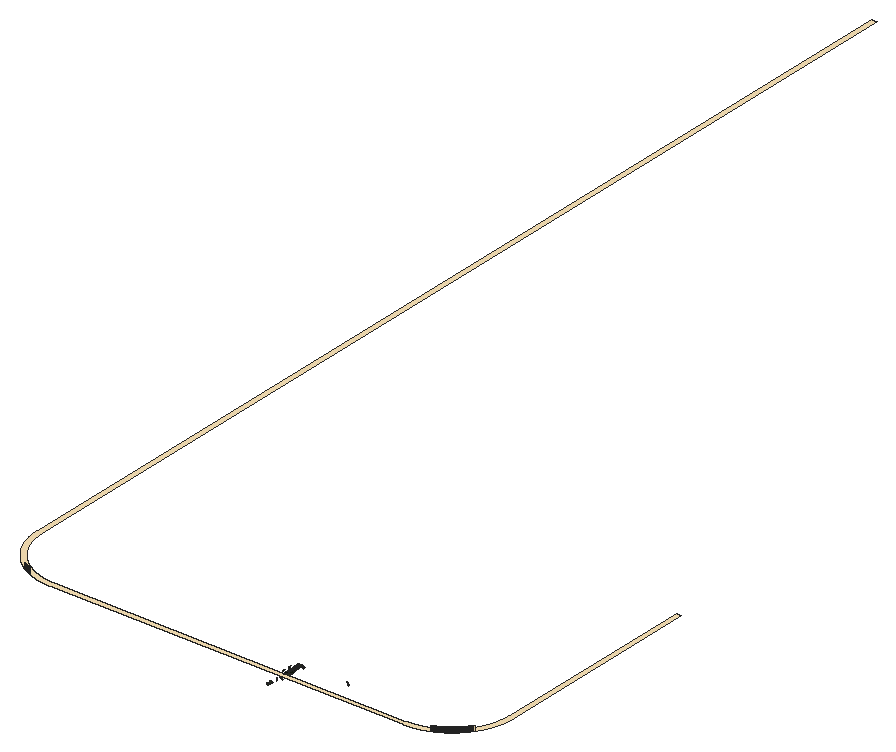
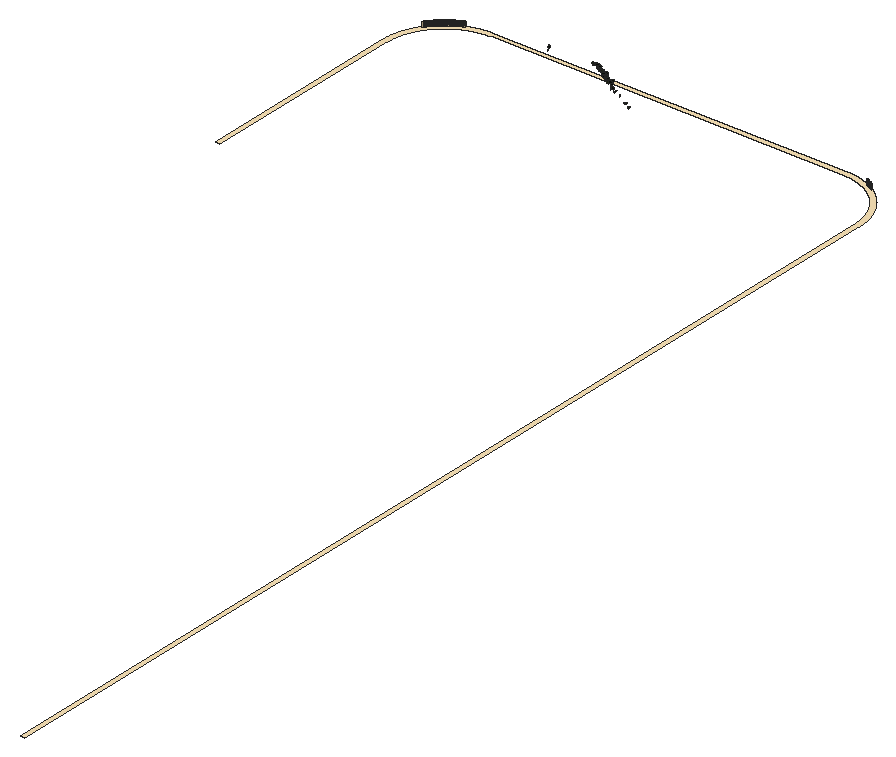
# SketchUp Ruby script. Lengths in inches.
U = 1.inch
M = Sketchup.active_model
def pt(a) = Geom::Point3d.new(a.map { |v| v * U })
def face(e, loops, mat)
  f = e.add_face(loops[0].map { |a| pt(a) })
  loops[1..].each { |l| e.add_face(l.map { |a| pt(a) }).erase! }
  f.material = f.back_material = mat if mat
  f
end
# faces: each face lists its corners as indices into pts; further lists are holes
def faces(e, pts, list, mat = nil) = list.each { |f| face(e, (f[0].is_a?(Array) ? f : [f]).map { |l| l.map { |i| pts[i] } }, mat) }
# xy, xz, yz: faces in a plane at the given z, y or x. An outline is a flat list of corners, or four numbers for a rectangle; further outlines are holes
def ring(l) = l.size == 4 ? [[l[0], l[1]], [l[2], l[1]], [l[2], l[3]], [l[0], l[3]]] : l.each_slice(2).to_a
def flat(e, list, mat, &to3) = list.each { |f| face(e, (f[0].is_a?(Array) ? f : [f]).map { |l| ring(l).map { |u, v| to3.(u, v) } }, mat) }
def xy(e, z, list, mat = nil) = flat(e, list, mat) { |x, y| [x, y, z] }
def xz(e, y, list, mat = nil) = flat(e, list, mat) { |x, z| [x, y, z] }
def yz(e, x, list, mat = nil) = flat(e, list, mat) { |y, z| [x, y, z] }
def lines(e, pts, list) = list.each { |a, b| e.add_line(pt(pts[a]), pt(pts[b])) }
# prism: a flat outline (further loops are holes) pulled along v
def prism(e, loops, v, mat = nil)
  f = face(e, loops, mat); d = Geom::Vector3d.new(v.map { |x| x * U })
  f.pushpull(f.normal.samedirection?(d) ? d.length : -d.length)
end
def box(e, o, s, mat = nil) = prism(e, [[o, [o[0] + s[0], o[1], o[2]], [o[0] + s[0], o[1] + s[1], o[2]], [o[0], o[1] + s[1], o[2]]]], [0, 0, s[2]], mat)
def at(x, y, z, deg = 0) = Geom::Transformation.translation(pt([x, y, z])) * Geom::Transformation.rotation(ORIGIN, Z_AXIS, deg.degrees)
def axes(o, x, y, z) = Geom::Transformation.new([*x, 0, *y, 0, *z, 0, *pt(o).to_a, 1])
def part(name) = M.definitions.add(name)
# library, detail: a bought-in or finely detailed component or shape, given as its bounding box
def library(name, o, s) = part(name).tap { |d| box(d.entities, o, s) }
def detail(e, o, s) = box(e.add_group.entities, o, s)
def put(e, d, t, mat = nil) = e.add_instance(d, t).tap { |i| i.material = mat if mat }
def group(e, t, mat = nil) = e.add_group.tap { |g| g.transformation = t; g.material = mat if mat }.entities
root = M.entities
M.materials.add("1026 AP 7946 SUNNY SIDE UP").color = [254, 231, 186]
M.materials.add("efeu1").color = [18, 25, 13]
M.materials.add("efeu2").color = [43, 57, 29]
c1 = part("ivyleaf_10")
p = [[0,0.5,-0.03],[-0.0625,2.02,-0.43],[-0.19,2.01,-0.46],[-0.54,1.05,-0.29],[-0.52,0.625,-0.18],[-0.83,0.76,-0.28],
  [-1.16,0.64,-0.33],[-1.15,0.33,-0.24],[-0.77,-0.39,0.02],[-0.3,-0.51,0.16],[0.04,-0.48,0.23],[-0.02,2.01,-0.4375],
  [-0.06,2.01,-0.43],[0.04,-0.49,0.23],[0.67,-0.49,0.14],[1.38,0.36,-0.2],[1.375,0.51,-0.24],[0.81,0.65,-0.19],
  [0.62,0.59,-0.15],[0.6,1.09,-0.28],[0.5,1.23,-0.31]]
faces(c1.entities,p,[[0,1,2,3,4,5,6,7,8,9,10],[11,12,0,13,14,15,16,17,18,19,20]],"efeu2")
c2 = part("ivyleaf_9")
p = [[1.54,2.16,1.25],[1.36,2.04,1.19],[-0.21,0.99,0.68],[-0.71,1.11,0.82],[-0.85,0.86,0.67],[-0.8,0.17,0.21],
  [-0.9,-0.01,0.1],[-0.67,-0.16,-0.02],[-0.08,-0.08,-0.05],[-0.03,-0.6,-0.4],[0.65,-0.88,-0.66],[0.83,-0.6,-0.49],
  [1.29,-0.42,-0.43],[1.8125,-0.07,-0.26],[1.21,0.44,0.15]]
faces(c2.entities,p,[[0,1,2,3,4,5,6,7,8,9,10,11,12,13,14]],"efeu1")
xy(root,274,[[177,213,29.75,213.001,29.728,213.001,29.645,213.003,29.49,213.005,29.472,213.005,29.455,213.006,29.365,213.008,29.234,213.011,29.208,213.012,29.183,213.013,29.094,213.016,28.979,213.02,28.944,213.022,28.911,213.023,28.827,213.027,28.724,213.031,28.68,213.034,28.639,213.036,28.561,213.04,28.469,213.045,28.416,213.048,28.367,213.051,28.296,213.056,28.215,213.061,28.152,213.066,28.096,213.07,28.032,213.075,27.96,213.08,27.888,213.086,27.824,213.091,27.768,213.096,27.706,213.101,27.624,213.109,27.553,213.115,27.505,213.12,27.452,213.125,27.36,213.135,27.282,213.142,27.242,213.147,27.198,213.151,27.095,213.163,27.012,213.172,26.979,213.176,26.944,213.18,26.83,213.194,26.741,213.205,26.717,213.208,26.691,213.211,26.561,213.229,26.471,213.241,26.455,213.243,26.4375,213.245,26.284,213.267,26.202,213.279,26.193,213.28,26.185,213.281,25.933,213.32,25.681,213.361,25.672,213.363,25.664,213.364,25.582,213.378,25.412,213.408,25.396,213.411,25.307,213.427,25.178,213.451,25.128,213.461,25.041,213.478,24.928,213.5,24.893,213.507,24.861,213.513,24.778,213.53,24.678,213.551,24.634,213.56,24.594,213.568,24.518,213.585,24.428,213.604,24.376,213.616,24.328,213.626,24.259,213.642,24.179,213.66,24.118,213.674,24.063,213.687,24,213.702,23.93,213.718,23.861,213.735,23.798,213.75,23.743,213.764,23.603,213.799,23.534,213.817,23.487,213.829,23.435,213.842,23.346,213.866,23.271,213.886,23.231,213.897,23.189,213.908,23.089,213.935,23.008,213.958,22.976,213.967,22.943,213.976,22.832,214.008,22.746,214.032,22.722,214.039,22.697,214.047,22.572,214.084,22.485,214.11,22.453,214.12,22.304,214.165,22.225,214.19,22.217,214.192,22.209,214.195,21.966,214.273,21.723,214.353,21.715,214.355,21.707,214.358,21.629,214.385,21.482,214.435,21.465,214.441,21.449,214.446,21.364,214.476,21.241,214.52,21.216,214.529,21.193,214.537,21.109,214.568,21.001,214.607,20.968,214.619,20.937,214.631,20.858,214.66,20.762,214.697,20.721,214.712,20.682,214.727,20.609,214.755,20.524,214.788,20.429,214.826,20.362,214.852,20.287,214.883,20.229,214.906,20.176,214.927,20.117,214.952,20.05,214.979,19.984,215.007,19.925,215.032,19.872,215.054,19.815,215.078,19.74,215.11,19.674,215.138,19.629,215.158,19.581,215.179,19.497,215.216,19.425,215.248,19.387,215.265,19.347,215.283,19.254,215.325,19.177,215.36,19.147,215.374,19.115,215.388,19.01,215.437,18.93,215.474,18.884,215.496,18.766,215.553,18.684,215.592,18.669,215.599,18.653,215.607,18.514,215.675,18.439,215.711,18.432,215.715,18.424,215.719,18.196,215.834,17.969,215.951,17.962,215.955,17.954,215.959,17.881,215.997,17.744,216.07,17.728,216.078,17.714,216.086,17.634,216.129,17.519,216.191,17.496,216.204,17.474,216.216,17.397,216.259,17.296,216.315,17.265,216.332,17.236,216.348,17.163,216.39,17.074,216.441,17.036,216.463,17,216.483,16.932,216.523,16.853,216.569,16.807,216.596,16.765,216.621,16.704,216.657,16.633,216.699,16.58,216.731,16.531,216.761,16.477,216.794,16.415,216.831,16.354,216.869,16.299,216.903,16.251,216.933,16.198,216.966,16.129,217.009,16.068,217.047,16.027,217.074,15.982,217.102,15.905,217.152,15.839,217.195,15.805,217.217,15.768,217.241,15.682,217.298,15.612,217.344,15.584,217.362,15.555,217.382,15.46,217.446,15.386,217.496,15.365,217.51,15.344,217.525,15.236,217.599,15.161,217.65,15.148,217.66,15.133,217.67,15.006,217.759,14.939,217.807,14.925,217.817,14.718,217.966,14.512,218.117,14.498,218.127,14.432,218.176,14.308,218.27,14.28,218.29,14.209,218.345,14.105,218.425,14.084,218.441,14.064,218.456,13.994,218.511,13.904,218.582,13.876,218.604,13.85,218.624,13.784,218.677,13.704,218.741,13.67,218.769,13.638,218.794,13.577,218.844,13.506,218.902,13.465,218.936,13.427,218.967,13.372,219.012,13.309,219.065,13.262,219.105,13.218,219.141,13.169,219.183,13.114,219.229,13.06,219.276,13.011,219.318,12.968,219.355,12.921,219.396,12.86,219.45,12.806,219.497,12.769,219.53,12.729,219.565,12.661,219.626,12.603,219.678,12.572,219.706,12.539,219.735,12.464,219.805,12.401,219.861,12.377,219.884,12.351,219.908,12.267,219.986,12.202,220.047,12.184,220.064,12.07,220.172,12.004,220.234,11.98,220.258,11.868,220.366,11.809,220.424,11.797,220.436,11.615,220.615,11.436,220.797,11.424,220.809,11.366,220.868,11.258,220.98,11.234,221.004,11.172,221.07,11.064,221.184,11.047,221.202,10.986,221.267,10.908,221.351,10.884,221.377,10.861,221.401,10.805,221.464,10.735,221.539,10.706,221.572,10.678,221.603,10.626,221.661,10.565,221.729,10.53,221.769,10.497,221.806,10.45,221.86,10.396,221.921,10.355,221.968,10.318,222.011,10.276,222.06,10.229,222.114,10.183,222.169,10.141,222.218,10.105,222.262,10.065,222.309,10.012,222.372,9.967,222.427,9.936,222.465,9.902,222.506,9.844,222.577,9.794,222.638,9.769,222.67,9.741,222.704,9.677,222.784,9.624,222.85,9.604,222.876,9.582,222.904,9.511,222.994,9.456,223.064,9.441,223.084,9.425,223.105,9.345,223.209,9.29,223.28,9.27,223.308,9.176,223.432,9.127,223.498,9.117,223.512,8.966,223.718,8.817,223.925,8.807,223.939,8.759,224.006,8.67,224.133,8.66,224.148,8.65,224.161,8.599,224.236,8.525,224.344,8.51,224.365,8.496,224.386,8.446,224.46,8.382,224.555,8.362,224.584,8.344,224.612,8.298,224.682,8.241,224.768,8.217,224.805,8.195,224.839,8.152,224.905,8.102,224.982,8.074,225.027,8.047,225.068,8.009,225.129,7.966,225.198,7.933,225.251,7.903,225.299,7.869,225.354,7.831,225.415,7.794,225.477,7.761,225.531,7.731,225.58,7.699,225.633,7.657,225.704,7.621,225.765,7.596,225.807,7.569,225.853,7.523,225.932,7.483,226,7.463,226.036,7.441,226.074,7.39,226.163,7.348,226.236,7.332,226.265,7.315,226.296,7.259,226.397,7.216,226.474,7.204,226.496,7.191,226.519,7.129,226.634,7.086,226.714,7.078,226.728,7.07,226.744,6.997,226.881,6.959,226.954,6.955,226.962,6.951,226.969,6.834,227.196,6.719,227.424,6.715,227.432,6.711,227.439,6.675,227.514,6.607,227.653,6.599,227.669,6.592,227.684,6.553,227.766,6.496,227.884,6.474,227.93,6.437,228.01,6.388,228.115,6.374,228.147,6.36,228.177,6.325,228.254,6.283,228.347,6.265,228.387,6.248,228.425,6.216,228.497,6.179,228.581,6.158,228.629,6.138,228.674,6.11,228.74,6.078,228.815,6.054,228.872,6.032,228.925,6.007,228.984,5.979,229.05,5.952,229.117,5.927,229.176,5.906,229.229,5.883,229.287,5.852,229.362,5.826,229.429,5.788,229.524,5.755,229.609,5.727,229.682,5.712,229.721,5.697,229.762,5.66,229.858,5.631,229.937,5.619,229.968,5.607,230.001,5.568,230.109,5.537,230.193,5.529,230.216,5.52,230.241,5.476,230.364,5.446,230.449,5.441,230.465,5.435,230.482,5.385,230.629,5.358,230.707,5.355,230.715,5.353,230.723,5.273,230.966,5.195,231.209,5.192,231.217,5.19,231.225,5.165,231.304,5.12,231.453,5.11,231.485,5.084,231.572,5.047,231.697,5.039,231.722,5.032,231.746,5.008,231.832,4.976,231.943,4.967,231.976,4.958,232.008,4.935,232.089,4.908,232.189,4.897,232.231,4.886,232.271,4.866,232.346,4.842,232.435,4.829,232.487,4.817,232.534,4.799,232.603,4.764,232.743,4.75,232.798,4.735,232.861,4.718,232.93,4.702,233,4.687,233.063,4.674,233.118,4.66,233.179,4.642,233.259,4.626,233.328,4.616,233.376,4.604,233.428,4.585,233.518,4.568,233.594,4.56,233.634,4.551,233.678,4.53,233.778,4.513,233.861,4.507,233.893,4.5,233.928,4.478,234.041,4.461,234.128,4.451,234.178,4.427,234.307,4.411,234.396,4.408,234.412,4.378,234.582,4.364,234.664,4.363,234.672,4.361,234.681,4.32,234.933,4.281,235.185,4.28,235.193,4.279,235.202,4.267,235.284,4.245,235.4375,4.243,235.455,4.241,235.471,4.229,235.561,4.211,235.691,4.208,235.717,4.205,235.741,4.194,235.83,4.18,235.944,4.176,235.979,4.172,236.012,4.163,236.095,4.151,236.198,4.147,236.242,4.142,236.282,4.135,236.36,4.125,236.452,4.12,236.505,4.115,236.553,4.109,236.624,4.101,236.706,4.096,236.768,4.091,236.824,4.086,236.888,4.08,236.96,4.075,237.032,4.07,237.096,4.066,237.152,4.061,237.215,4.056,237.296,4.051,237.367,4.048,237.416,4.045,237.469,4.04,237.561,4.036,237.639,4.034,237.68,4.031,237.724,4.027,237.827,4.023,237.911,4.022,237.944,4.02,237.979,4.016,238.094,4.013,238.183,4.012,238.208,4.011,238.234,4.008,238.365,4.006,238.455,4.005,238.472,4.005,238.49,4.003,238.645,4.001,238.728,4.001,238.745,4,238.995,4,674,6,674,6,239,6.001,238.764,6.001,238.749,6.002,238.675,6.005,238.529,6.005,238.497,6.007,238.416,6.01,238.293,6.011,238.269,6.012,238.246,6.015,238.165,6.019,238.058,6.02,238.025,6.021,237.995,6.025,237.918,6.029,237.822,6.031,237.781,6.033,237.744,6.037,237.673,6.042,237.587,6.045,237.538,6.047,237.493,6.052,237.428,6.057,237.352,6.061,237.294,6.064,237.242,6.069,237.184,6.074,237.117,6.08,237.05,6.084,236.992,6.089,236.94,6.094,236.882,6.101,236.806,6.107,236.741,6.111,236.697,6.116,236.648,6.124,236.5625,6.131,236.491,6.136,236.454,6.14,236.413,6.151,236.318,6.159,236.242,6.163,236.212,6.166,236.179,6.18,236.072,6.189,235.992,6.192,235.97,6.195,235.945,6.211,235.824,6.222,235.743,6.224,235.728,6.226,235.712,6.247,235.567,6.257,235.494,6.259,235.487,6.26,235.478,6.295,235.246,6.333,235.013,6.335,235.005,6.336,234.998,6.349,234.925,6.374,234.781,6.377,234.765,6.379,234.75,6.394,234.67,6.416,234.549,6.421,234.525,6.425,234.503,6.441,234.424,6.461,234.318,6.468,234.286,6.473,234.256,6.489,234.181,6.508,234.087,6.517,234.047,6.524,234.01,6.54,233.94,6.558,233.857,6.568,233.808,6.578,233.765,6.593,233.701,6.609,233.627,6.623,233.57,6.634,233.52,6.648,233.463,6.663,233.397,6.679,233.332,6.693,233.275,6.705,233.225,6.719,233.168,6.738,233.095,6.754,233.031,6.765,232.988,6.778,232.94,6.8,232.857,6.818,232.788,6.828,232.752,6.838,232.713,6.864,232.62,6.884,232.546,6.892,232.517,6.901,232.485,6.931,232.382,6.953,232.304,6.959,232.283,6.966,232.259,7.001,232.142,7.024,232.063,7.029,232.049,7.033,232.033,7.077,231.893,7.098,231.823,7.101,231.816,7.103,231.808,7.175,231.584,7.249,231.36,7.251,231.352,7.254,231.345,7.277,231.276,7.325,231.137,7.335,231.107,7.362,231.03,7.403,230.915,7.411,230.892,7.419,230.87,7.447,230.794,7.483,230.693,7.495,230.662,7.505,230.634,7.532,230.5625,7.566,230.473,7.581,230.434,7.594,230.399,7.62,230.333,7.651,230.253,7.669,230.207,7.685,230.165,7.71,230.104,7.738,230.034,7.76,229.98,7.779,229.932,7.802,229.878,7.827,229.816,7.853,229.754,7.875,229.7,7.896,229.652,7.918,229.598,7.948,229.528,7.974,229.468,7.992,229.428,8.011,229.382,8.046,229.304,8.075,229.238,8.09,229.204,8.107,229.167,8.147,229.079,8.178,229.009,8.191,228.982,8.205,228.952,8.25,228.855,8.284,228.781,8.294,228.761,8.304,228.739,8.357,228.628,8.392,228.554,8.399,228.541,8.406,228.526,8.471,228.395,8.503,228.329,8.506,228.322,8.51,228.315,8.616,228.104,8.724,227.895,8.728,227.888,8.731,227.881,8.765,227.816,8.834,227.686,8.842,227.672,8.849,227.659,8.888,227.587,8.946,227.479,8.958,227.458,8.969,227.438,9.008,227.367,9.06,227.273,9.076,227.245,9.091,227.218,9.129,227.152,9.176,227.068,9.197,227.032,9.215,227,9.251,226.938,9.294,226.864,9.32,226.822,9.342,226.783,9.376,226.727,9.445,226.612,9.471,226.567,9.502,226.517,9.572,226.403,9.603,226.353,9.63,226.309,9.661,226.26,9.701,226.195,9.736,226.14,9.76,226.103,9.787,226.061,9.833,225.989,9.872,225.929,9.892,225.897,9.915,225.863,9.968,225.783,10.01,225.719,10.027,225.694,10.045,225.666,10.105,225.577,10.15,225.51,10.163,225.491,10.177,225.471,10.246,225.37,10.292,225.303,10.31,225.277,10.395,225.157,10.437,225.097,10.441,225.091,10.446,225.084,10.584,224.893,10.723,224.703,10.728,224.697,10.732,224.691,10.776,224.632,10.864,224.515,10.874,224.502,10.883,224.49,10.933,224.425,11.007,224.327,11.023,224.308,11.036,224.29,11.086,224.227,11.152,224.142,11.173,224.116,11.191,224.092,11.239,224.033,11.299,223.957,11.325,223.925,11.348,223.896,11.394,223.841,11.448,223.775,11.479,223.736,11.508,223.702,11.55,223.652,11.598,223.593,11.636,223.549,11.669,223.509,11.707,223.464,11.75,223.413,11.794,223.362,11.832,223.318,11.866,223.279,11.904,223.235,11.954,223.178,11.997,223.129,12.027,223.095,12.06,223.058,12.117,222.994,12.165,222.941,12.19,222.913,12.217,222.883,12.282,222.812,12.334,222.755,12.354,222.733,12.376,222.709,12.45,222.63,12.505,222.571,12.52,222.554,12.537,222.537,12.622,222.448,12.678,222.389,12.688,222.378,12.7,222.366,12.802,222.261,12.853,222.208,12.864,222.197,13.029,222.029,13.197,221.864,13.208,221.853,13.261,221.802,13.366,221.7,13.378,221.688,13.389,221.678,13.448,221.622,13.537,221.537,13.554,221.52,13.571,221.505,13.63,221.45,13.709,221.376,13.733,221.354,13.755,221.334,13.812,221.282,13.883,221.217,13.913,221.19,13.941,221.165,13.994,221.117,14.058,221.06,14.095,221.027,14.129,220.997,14.178,220.954,14.235,220.904,14.279,220.866,14.318,220.832,14.362,220.794,14.413,220.75,14.464,220.707,14.509,220.669,14.549,220.636,14.593,220.598,14.652,220.55,14.702,220.508,14.736,220.479,14.775,220.448,14.841,220.394,14.896,220.348,14.925,220.325,14.957,220.299,15.033,220.239,15.092,220.191,15.116,220.173,15.142,220.152,15.227,220.086,15.29,220.036,15.308,220.023,15.327,220.007,15.425,219.933,15.49,219.883,15.502,219.874,15.515,219.864,15.632,219.776,15.691,219.732,15.697,219.728,15.703,219.723,15.893,219.584,16.084,219.446,16.091,219.441,16.097,219.437,16.157,219.395,16.277,219.31,16.303,219.292,16.37,219.246,16.471,219.177,16.491,219.163,16.51,219.15,16.577,219.105,16.666,219.045,16.694,219.027,16.719,219.01,16.783,218.968,16.863,218.915,16.897,218.892,16.929,218.872,16.989,218.833,17.061,218.787,17.103,218.76,17.14,218.736,17.195,218.701,17.26,218.661,17.309,218.63,17.353,218.603,17.403,218.572,17.517,218.502,17.567,218.471,17.612,218.445,17.727,218.376,17.783,218.342,17.822,218.32,17.864,218.294,17.938,218.251,18,218.215,18.032,218.197,18.068,218.176,18.152,218.129,18.218,218.091,18.245,218.076,18.273,218.06,18.367,218.008,18.438,217.969,18.458,217.958,18.479,217.946,18.587,217.888,18.659,217.849,18.672,217.842,18.686,217.834,18.816,217.765,18.881,217.731,18.888,217.728,18.895,217.724,19.104,217.616,19.315,217.51,19.322,217.506,19.329,217.503,19.395,217.471,19.526,217.406,19.541,217.399,19.554,217.392,19.628,217.357,19.739,217.304,19.761,217.294,19.781,217.284,19.855,217.25,19.952,217.205,19.982,217.191,20.009,217.178,20.079,217.147,20.167,217.107,20.204,217.09,20.238,217.075,20.304,217.046,20.382,217.011,20.428,216.992,20.468,216.974,20.528,216.948,20.598,216.918,20.652,216.896,20.7,216.875,20.754,216.853,20.816,216.827,20.878,216.802,20.932,216.779,20.98,216.76,21.034,216.738,21.104,216.71,21.165,216.685,21.207,216.669,21.253,216.651,21.333,216.62,21.399,216.594,21.434,216.581,21.473,216.566,21.5625,216.532,21.634,216.505,21.662,216.495,21.693,216.483,21.794,216.447,21.87,216.419,21.892,216.411,21.915,216.403,22.03,216.362,22.107,216.335,22.137,216.325,22.276,216.277,22.345,216.254,22.352,216.251,22.36,216.249,22.584,216.175,22.808,216.103,22.816,216.101,22.823,216.098,22.893,216.077,23.033,216.033,23.049,216.029,23.063,216.024,23.142,216.001,23.259,215.966,23.283,215.959,23.304,215.953,23.382,215.931,23.485,215.901,23.517,215.892,23.546,215.884,23.62,215.864,23.713,215.838,23.752,215.828,23.788,215.818,23.857,215.8,23.94,215.778,23.988,215.765,24.031,215.754,24.095,215.738,24.168,215.719,24.225,215.705,24.275,215.693,24.332,215.679,24.397,215.663,24.463,215.648,24.52,215.634,24.57,215.623,24.627,215.609,24.701,215.593,24.765,215.578,24.808,215.568,24.857,215.558,24.94,215.54,25.01,215.524,25.047,215.517,25.087,215.508,25.181,215.489,25.256,215.473,25.286,215.468,25.318,215.461,25.424,215.441,25.503,215.425,25.525,215.421,25.549,215.416,25.67,215.394,25.75,215.379,25.765,215.377,25.781,215.374,25.925,215.349,25.998,215.336,26.005,215.335,26.013,215.333,26.246,215.295,26.478,215.26,26.487,215.259,26.494,215.257,26.567,215.247,26.712,215.226,26.728,215.224,26.743,215.222,26.824,215.211,26.945,215.195,26.97,215.192,26.992,215.189,27.072,215.18,27.179,215.166,27.212,215.163,27.242,215.159,27.318,215.151,27.413,215.14,27.454,215.136,27.491,215.131,27.5625,215.124,27.648,215.116,27.697,215.111,27.741,215.107,27.806,215.101,27.882,215.094,27.94,215.089,27.992,215.084,28.05,215.08,28.117,215.074,28.184,215.069,28.242,215.064,28.294,215.061,28.352,215.057,28.428,215.052,28.493,215.047,28.538,215.045,28.587,215.042,28.673,215.037,28.744,215.033,28.781,215.031,28.822,215.029,28.918,215.025,28.995,215.021,29.025,215.02,29.058,215.019,29.165,215.015,29.246,215.012,29.269,215.011,29.293,215.01,29.416,215.007,29.497,215.005,29.529,215.005,29.675,215.002,29.749,215.001,29.764,215.001,177,215,177.251,215.001,177.503,215.005,177.754,215.012,178.005,215.021,178.256,215.033,178.507,215.047,178.758,215.064,179.008,215.084,179.259,215.107,179.509,215.131,179.758,215.159,180.008,215.189,180.257,215.222,180.506,215.257,180.754,215.295,181.002,215.336,181.25,215.379,181.497,215.425,181.744,215.473,181.99,215.524,182.235,215.578,182.48,215.634,182.725,215.693,182.969,215.754,183.212,215.818,183.454,215.884,183.696,215.953,183.937,216.024,184.177,216.098,184.416,216.175,184.655,216.254,184.893,216.335,185.13,216.419,185.366,216.505,185.601,216.594,185.835,216.685,186.068,216.779,186.3,216.875,186.532,216.974,186.762,217.075,186.991,217.178,187.219,217.284,187.446,217.392,187.671,217.503,187.896,217.616,188.119,217.731,188.341,217.849,188.562,217.969,188.782,218.091,189,218.215,189.217,218.342,189.433,218.471,189.647,218.603,189.86,218.736,190.071,218.872,190.281,219.01,190.49,219.15,190.697,219.292,190.903,219.437,191.107,219.584,191.309,219.732,191.51,219.883,191.71,220.036,191.908,220.191,192.104,220.348,192.298,220.508,192.491,220.669,192.682,220.832,192.871,220.997,193.059,221.165,193.245,221.334,193.429,221.505,193.611,221.678,193.792,221.853,193.971,222.029,194.147,222.208,194.322,222.389,194.495,222.571,194.666,222.755,194.835,222.941,195.003,223.129,195.168,223.318,195.331,223.509,195.492,223.702,195.652,223.896,195.809,224.092,195.964,224.29,196.117,224.49,196.268,224.691,196.416,224.893,196.563,225.097,196.708,225.303,196.85,225.51,196.99,225.719,197.128,225.929,197.264,226.14,197.397,226.353,197.529,226.567,197.658,226.783,197.785,227,197.909,227.218,198.031,227.438,198.151,227.659,198.269,227.881,198.384,228.104,198.497,228.329,198.608,228.554,198.716,228.781,198.822,229.009,198.925,229.238,199.026,229.468,199.125,229.7,199.221,229.932,199.315,230.165,199.406,230.399,199.495,230.634,199.581,230.87,199.665,231.107,199.746,231.345,199.825,231.584,199.902,231.823,199.976,232.063,200.047,232.304,200.116,232.546,200.182,232.788,200.246,233.031,200.307,233.275,200.366,233.52,200.422,233.765,200.476,234.01,200.527,234.256,200.575,234.503,200.621,234.75,200.664,234.998,200.705,235.246,200.743,235.494,200.778,235.743,200.811,235.992,200.841,236.242,200.869,236.491,200.893,236.741,200.916,236.992,200.936,237.242,200.953,237.493,200.967,237.744,200.979,237.995,200.988,238.246,200.995,238.497,200.999,238.749,201,239,201,326,203,326,203,239,202.999,238.728,202.994,238.455,202.987,238.183,202.977,237.911,202.964,237.639,202.949,237.367,202.93,237.096,202.909,236.824,202.885,236.553,202.858,236.282,202.828,236.012,202.795,235.741,202.759,235.471,202.721,235.202,202.68,234.933,202.636,234.664,202.589,234.396,202.539,234.128,202.487,233.861,202.432,233.594,202.374,233.328,202.313,233.063,202.249,232.798,202.183,232.534,202.114,232.271,202.042,232.008,201.968,231.746,201.89,231.485,201.81,231.225,201.727,230.966,201.642,230.707,201.554,230.449,201.463,230.193,201.369,229.937,201.273,229.682,201.174,229.429,201.073,229.176,200.968,228.925,200.862,228.674,200.752,228.425,200.64,228.177,200.526,227.93,200.408,227.684,200.289,227.439,200.166,227.196,200.041,226.954,199.914,226.714,199.784,226.474,199.652,226.237,199.517,226,199.379,225.765,199.239,225.531,199.097,225.299,198.953,225.069,198.805,224.839,198.656,224.612,198.504,224.386,198.35,224.161,198.193,223.939,198.034,223.718,197.873,223.498,197.71,223.28,197.544,223.064,197.376,222.85,197.206,222.638,197.033,222.427,196.859,222.218,196.682,222.011,196.503,221.806,196.322,221.603,196.139,221.401,195.953,221.202,195.766,221.004,195.576,220.809,195.385,220.615,195.191,220.424,194.996,220.234,194.798,220.047,194.599,219.861,194.397,219.678,194.194,219.497,193.989,219.318,193.782,219.141,193.573,218.967,193.362,218.794,193.15,218.624,192.936,218.456,192.72,218.29,192.502,218.127,192.282,217.966,192.061,217.807,191.839,217.65,191.614,217.496,191.388,217.344,191.161,217.195,190.931,217.047,190.701,216.903,190.469,216.761,190.235,216.621,190,216.483,189.763,216.348,189.526,216.216,189.286,216.086,189.046,215.959,188.804,215.834,188.561,215.711,188.316,215.592,188.07,215.474,187.823,215.36,187.575,215.248,187.326,215.138,187.075,215.032,186.824,214.927,186.571,214.826,186.318,214.727,186.063,214.631,185.807,214.537,185.551,214.446,185.293,214.358,185.034,214.273,184.775,214.19,184.515,214.11,184.254,214.032,183.992,213.958,183.729,213.886,183.466,213.817,183.202,213.751,182.937,213.687,182.672,213.626,182.406,213.568,182.139,213.513,181.872,213.461,181.604,213.411,181.336,213.364,181.067,213.32,180.798,213.279,180.529,213.241,180.259,213.205,179.988,213.172,179.718,213.142,179.447,213.115,179.176,213.091,178.904,213.07,178.633,213.051,178.361,213.036,178.089,213.023,177.817,213.013,177.545,213.006,177.272,213.001]],"1026 AP 7946 SUNNY SIDE UP")
p = [[187.326,215.138,276],[187.075,215.032,276],[187.075,215.032,274],[187.326,215.138,274],[19.674,215.138,276],[19.629,215.158,276],
  [19.629,215.158,274],[19.674,215.138,274],[19.74,215.11,276],[19.74,215.11,274],[19.815,215.078,276],[19.815,215.078,274],
  [19.872,215.054,276],[19.872,215.054,274],[187.575,215.248,276],[187.575,215.248,274],[19.425,215.248,276],[19.387,215.265,276],
  [19.387,215.265,274],[19.425,215.248,274],[19.497,215.216,276],[19.497,215.216,274],[19.581,215.179,276],[19.581,215.179,274],
  [187.823,215.36,276],[187.823,215.36,274],[19.254,215.325,276],[19.177,215.36,276],[19.177,215.36,274],[19.254,215.325,274],
  [19.347,215.283,276],[19.347,215.283,274],[19.01,215.437,276],[18.93,215.474,276],[18.93,215.474,274],[19.01,215.437,274],
  [19.115,215.388,276],[19.115,215.388,274],[19.147,215.374,276],[19.147,215.374,274],[188.07,215.474,276],[188.07,215.474,274],
  [18.884,215.496,276],[18.766,215.553,276],[18.766,215.553,274],[18.884,215.496,274],[18.907,215.485,276],[18.907,215.485,274],
  [188.316,215.592,276],[188.316,215.592,274],[18.653,215.607,276],[18.514,215.675,276],[18.514,215.675,274],[18.653,215.607,274],
  [18.669,215.599,276],[18.669,215.599,274],[18.684,215.592,276],[18.684,215.592,274],[188.561,215.711,276],[188.561,215.711,274],
  [18.424,215.719,276],[18.196,215.834,276],[18.196,215.834,274],[18.424,215.719,274],[18.432,215.715,276],[18.432,215.715,274],
  [18.439,215.711,276],[18.439,215.711,274],[188.804,215.834,276],[188.804,215.834,274],[17.969,215.951,276],[17.969,215.951,274],
  [189.046,215.959,276],[189.046,215.959,274],[17.881,215.997,276],[17.744,216.07,276],[17.744,216.07,274],[17.881,215.997,274],
  [17.954,215.959,276],[17.954,215.959,274],[17.962,215.955,276],[17.962,215.955,274],[189.286,216.086,276],[189.286,216.086,274],
  [17.634,216.129,276],[17.519,216.191,276],[17.519,216.191,274],[17.634,216.129,274],[17.714,216.086,276],[17.714,216.086,274],
  [17.728,216.078,276],[17.728,216.078,274],[189.526,216.216,276],[189.526,216.216,274],[17.474,216.216,276],[17.397,216.259,276],
  [17.397,216.259,274],[17.474,216.216,274],[17.496,216.204,276],[17.496,216.204,274],[189.763,216.348,276],[189.763,216.348,274],
  [17.236,216.348,276],[17.163,216.39,276],[17.163,216.39,274],[17.236,216.348,274],[17.265,216.332,276],[17.265,216.332,274],
  [17.296,216.315,276],[17.296,216.315,274],[190,216.483,276],[190,216.483,274],[17.074,216.441,276],[17.036,216.463,276],
  [17.036,216.463,274],[17.074,216.441,274],[16.932,216.523,276],[16.853,216.569,276],[16.853,216.569,274],[16.932,216.523,274],
  [17,216.483,276],[17,216.483,274],[190.235,216.621,276],[190.235,216.621,274],[16.765,216.621,276],[16.704,216.657,276],
  [16.704,216.657,274],[16.765,216.621,274],[16.807,216.596,276],[16.807,216.596,274],[190.469,216.761,276],[190.469,216.761,274],
  [16.58,216.731,276],[16.531,216.761,276],[16.531,216.761,274],[16.58,216.731,274],[16.633,216.699,276],[16.633,216.699,274],
  [16.415,216.831,276],[16.354,216.869,276],[16.354,216.869,274],[16.415,216.831,274],[16.477,216.794,276],[16.477,216.794,274],
  [190.701,216.903,276],[190.701,216.903,274],[16.251,216.933,276],[16.198,216.966,276],[16.198,216.966,274],[16.251,216.933,274],
  [16.299,216.903,276],[16.299,216.903,274],[190.931,217.047,276],[190.931,217.047,274],[16.129,217.009,276],[16.068,217.047,276],
  [16.068,217.047,274],[16.129,217.009,274],[191.161,217.195,276],[191.161,217.195,274],[191.388,217.344,276],[191.388,217.344,274],
  [191.614,217.496,276],[191.614,217.496,274],[191.839,217.65,276],[191.839,217.65,274],[192.061,217.807,276],[192.061,217.807,274],
  [192.282,217.966,276],[192.282,217.966,274],[192.502,218.127,276],[192.502,218.127,274],[192.72,218.29,276],[192.72,218.29,274],
  [192.936,218.456,276],[192.936,218.456,274],[193.15,218.624,276],[193.15,218.624,274],[193.362,218.794,276],[193.362,218.794,274],
  [193.573,218.967,276],[193.573,218.967,274],[193.782,219.141,276],[193.782,219.141,274],[193.989,219.318,276],[193.989,219.318,274],
  [194.194,219.497,276],[194.194,219.497,274],[194.397,219.678,276],[194.397,219.678,274],[194.599,219.861,276],[194.599,219.861,274],
  [194.798,220.047,276],[194.798,220.047,274],[194.996,220.234,276],[194.996,220.234,274],[195.191,220.424,276],[195.191,220.424,274],
  [195.385,220.615,276],[195.385,220.615,274],[195.576,220.809,276],[195.576,220.809,274],[195.766,221.004,276],[195.766,221.004,274],
  [195.953,221.202,276],[195.953,221.202,274],[196.139,221.401,276],[196.139,221.401,274],[196.322,221.603,276],[196.322,221.603,274],
  [196.503,221.806,276],[196.503,221.806,274],[196.682,222.011,276],[196.682,222.011,274],[196.859,222.218,276],[196.859,222.218,274],
  [197.033,222.427,276],[197.033,222.427,274],[197.206,222.638,276],[197.206,222.638,274],[197.376,222.85,276],[197.376,222.85,274],
  [197.544,223.064,276],[197.544,223.064,274],[197.71,223.28,276],[197.71,223.28,274],[197.873,223.498,276],[197.873,223.498,274],
  [198.034,223.718,276],[198.034,223.718,274],[198.193,223.939,276],[198.193,223.939,274],[198.35,224.161,276],[198.35,224.161,274]]
faces(root,p,[[0,1,2,3],[4,5,6,7],[8,4,7,9],[10,8,9,11],[12,10,11,13],[14,0,3,15],[16,17,18,19],[20,16,19,21],
  [22,20,21,23],[5,22,23,6],[24,14,15,25],[26,27,28,29],[30,26,29,31],[17,30,31,18],[32,33,34,35],[36,32,35,37],
  [38,36,37,39],[27,38,39,28],[40,24,25,41],[42,43,44,45],[46,42,45,47],[33,46,47,34],[48,40,41,49],[50,51,52,53],
  [54,50,53,55],[56,54,55,57],[43,56,57,44],[58,48,49,59],[60,61,62,63],[64,60,63,65],[66,64,65,67],[51,66,67,52],
  [68,58,59,69],[61,70,71,62],[72,68,69,73],[74,75,76,77],[78,74,77,79],[80,78,79,81],[70,80,81,71],[82,72,73,83],
  [84,85,86,87],[88,84,87,89],[90,88,89,91],[75,90,91,76],[92,82,83,93],[94,95,96,97],[98,94,97,99],[85,98,99,86],
  [100,92,93,101],[102,103,104,105],[106,102,105,107],[108,106,107,109],[95,108,109,96],[110,100,101,111],[112,113,114,115],[103,112,115,104],
  [116,117,118,119],[120,116,119,121],[113,120,121,114],[122,110,111,123],[124,125,126,127],[128,124,127,129],[117,128,129,118],[130,122,123,131],
  [132,133,134,135],[136,132,135,137],[125,136,137,126],[138,139,140,141],[142,138,141,143],[133,142,143,134],[144,130,131,145],[146,147,148,149],
  [150,146,149,151],[139,150,151,140],[152,144,145,153],[154,155,156,157],[147,154,157,148],[158,152,153,159],[160,158,159,161],[162,160,161,163],
  [164,162,163,165],[166,164,165,167],[168,166,167,169],[170,168,169,171],[172,170,171,173],[174,172,173,175],[176,174,175,177],[178,176,177,179],
  [180,178,179,181],[182,180,181,183],[184,182,183,185],[186,184,185,187],[188,186,187,189],[190,188,189,191],[192,190,191,193],[194,192,193,195],
  [196,194,195,197],[198,196,197,199],[200,198,199,201],[202,200,201,203],[204,202,203,205],[206,204,205,207],[208,206,207,209],[210,208,209,211],
  [212,210,211,213],[214,212,213,215],[216,214,215,217],[218,216,217,219],[220,218,219,221],[222,220,221,223],[224,222,223,225],[226,224,225,227],
  [228,226,227,229],[230,228,229,231],[232,230,231,233]],"1026 AP 7946 SUNNY SIDE UP")
put(root,c1,axes([119.14,215.05,267.875],[-0.41257,-0.02576,-0.03265],[0.0536,-0.02644,-0.27006],[0.03502,-0.26294,0.02878]),"1026 AP 7946 SUNNY SIDE UP")
put(root,c1,axes([120.36,215.09,268.95],[0.36849,0.13604,-0.00275],[0.00754,-0.0151,-0.27879],[-0.21385,0.23388,-0.01456]),"1026 AP 7946 SUNNY SIDE UP")
put(root,c1,axes([122.79,215.16,270.87],[-0.27672,0.21845,0.01277],[-0.045,-0.0088,-0.28762],[-0.34098,-0.17612,0.02759]),"1026 AP 7946 SUNNY SIDE UP")
put(root,c2,axes([124.34,215.26,272],[0.2643,-0.22869,-0.03842],[-0.00934,0.04021,-0.2915],[0.3639,0.16713,0.02043]),"1026 AP 7946 SUNNY SIDE UP")
put(root,c2,axes([125.53,215.38,272.94],[0.24494,0.21374,0.12536],[0.11546,0.09555,-0.27189],[-0.36811,0.17219,-0.00186]),"1026 AP 7946 SUNNY SIDE UP")
put(root,c2,axes([125.94,214.88,275.32],[0.0754,0.28185,0.06094],[-0.02963,0.0613,-0.29273],[-0.45136,0.04306,0.02939]),"1026 AP 7946 SUNNY SIDE UP")
put(root,c2,axes([125.88,215.27,272.87],[0.35375,-0.06489,-0.17835],[-0.24299,0.08264,-0.23882],[0.15859,0.27135,0.03191]),"1026 AP 7946 SUNNY SIDE UP")
put(root,c2,axes([126.34,215.01,274.18],[0.27011,0.22644,-0.02751],[-0.00524,-0.03254,-0.29248],[-0.35873,0.17098,-0.01644]),"1026 AP 7946 SUNNY SIDE UP")
put(root,c2,axes([126.73,215.05,274.73],[0.29313,0.21053,0.06693],[0.08916,0.03478,-0.28884],[-0.3342,0.19394,-0.01835]),"1026 AP 7946 SUNNY SIDE UP")
put(root,c2,axes([127.9,214.99,275.65],[0.35371,0.09494,0.18593],[0.16865,0.17261,-0.23095],[-0.27185,0.23062,0.09865]),"1026 AP 7946 SUNNY SIDE UP")
put(root,c1,axes([128.1,215.125,274.42],[0.44507,-0.05338,0.08366],[0.11804,-0.04019,-0.29588],[0.09767,0.2918,-0.02365]),"1026 AP 7946 SUNNY SIDE UP")
put(root,c2,axes([128.4375,214.95,277.36],[-0.07307,0.27934,0.1008],[-0.03222,0.09416,-0.29115],[-0.46347,-0.05059,0.00435]),"1026 AP 7946 SUNNY SIDE UP")
put(root,c1,axes([128.46,215.02,276.18],[-0.05831,0.30099,0.04141],[-0.01925,0.03726,-0.31211],[-0.47675,-0.03832,0.00754]),"1026 AP 7946 SUNNY SIDE UP")
put(root,c2,axes([128.41,215.11,276.3],[0.45767,0.00257,-0.04334],[-0.06537,-0.03119,-0.29839],[-0.011,0.29243,-0.02972]),"1026 AP 7946 SUNNY SIDE UP")
put(root,c2,axes([128.93,215.19,275.4],[-0.35838,-0.16186,-0.12386],[0.22024,0.00159,-0.27787],[0.22685,-0.25725,0.07411]),"1026 AP 7946 SUNNY SIDE UP")
put(root,c2,axes([129.56,215.27,275.9375],[-0.35338,-0.14459,0.15343],[-0.18056,-0.09771,-0.27528],[0.27301,-0.25177,0.01654]),"1026 AP 7946 SUNNY SIDE UP")
put(root,c2,axes([129.54,215.2,276.91],[-0.09592,-0.206,-0.21362],[0.20372,0.16953,-0.21299],[0.41053,-0.13226,0.05578]),"1026 AP 7946 SUNNY SIDE UP")
put(root,c1,axes([129.91,215.1,277.37],[-0.03121,0.171,0.25328],[-0.10625,0.23649,-0.17439],[-0.45747,-0.06659,0.02322]),"1026 AP 7946 SUNNY SIDE UP")
put(root,c1,axes([130.32,215.18,277.75],[-0.17115,-0.28064,0.08499],[-0.01024,-0.08737,-0.30957],[0.46056,-0.10623,0.0247]),"1026 AP 7946 SUNNY SIDE UP")
put(root,c2,axes([131.14,215.09,278.99],[-0.04976,0.30283,0.00009],[-0.08813,-0.00747,-0.30826],[-0.46795,-0.0308,0.05805]),"1026 AP 7946 SUNNY SIDE UP")
put(root,c1,axes([130.7,215.15,277.62],[0.27487,-0.11941,0.22057],[0.32243,-0.07438,-0.21497],[0.21295,0.26675,0.04079]),"1026 AP 7946 SUNNY SIDE UP")
put(root,c1,axes([131.07,215.16,277.8],[0.15485,0.23443,-0.16571],[-0.15078,-0.13435,-0.26083],[-0.42212,0.13399,0.03238]),"1026 AP 7946 SUNNY SIDE UP")
put(root,c1,axes([131.07,214.94,278.12],[0.24129,0.06138,0.27389],[0.24352,0.23108,-0.14589],[-0.35257,0.20161,0.08667]),"1026 AP 7946 SUNNY SIDE UP")
put(root,c2,axes([131.94,215.12,279.31],[0.15503,0.26546,-0.1176],[-0.06832,-0.10723,-0.29234],[-0.45016,0.1077,0.00387]),"1026 AP 7946 SUNNY SIDE UP")
put(root,c2,axes([131.9375,215.01,278.78],[0.3423,0.22304,0.05534],[0.0777,0.02494,-0.32041],[-0.3518,0.22253,-0.01693]),"1026 AP 7946 SUNNY SIDE UP")
put(root,c2,axes([132.13,215.21,279.33],[0.09145,-0.2997,0.02213],[0.03664,-0.01905,-0.31399],[0.47123,0.05964,0.02012]),"1026 AP 7946 SUNNY SIDE UP")
put(root,c1,axes([132.88,215.3,279.39],[-0.1464,-0.21197,0.20948],[-0.03975,-0.20798,-0.2351],[0.46146,-0.08516,0.04621]),"1026 AP 7946 SUNNY SIDE UP")
put(root,c1,axes([133.76,215.18,279.25],[-0.46133,0.1163,-0.0499],[0.05708,-0.04125,-0.32438],[-0.19011,-0.2946,0.0237]),"1026 AP 7946 SUNNY SIDE UP")
put(root,c2,axes([151.93,215.68,279.25],[0.41281,-0.17917,-0.33116],[-0.46311,0.13239,-0.32407],[0.34462,0.39252,-0.03882]),"1026 AP 7946 SUNNY SIDE UP")
